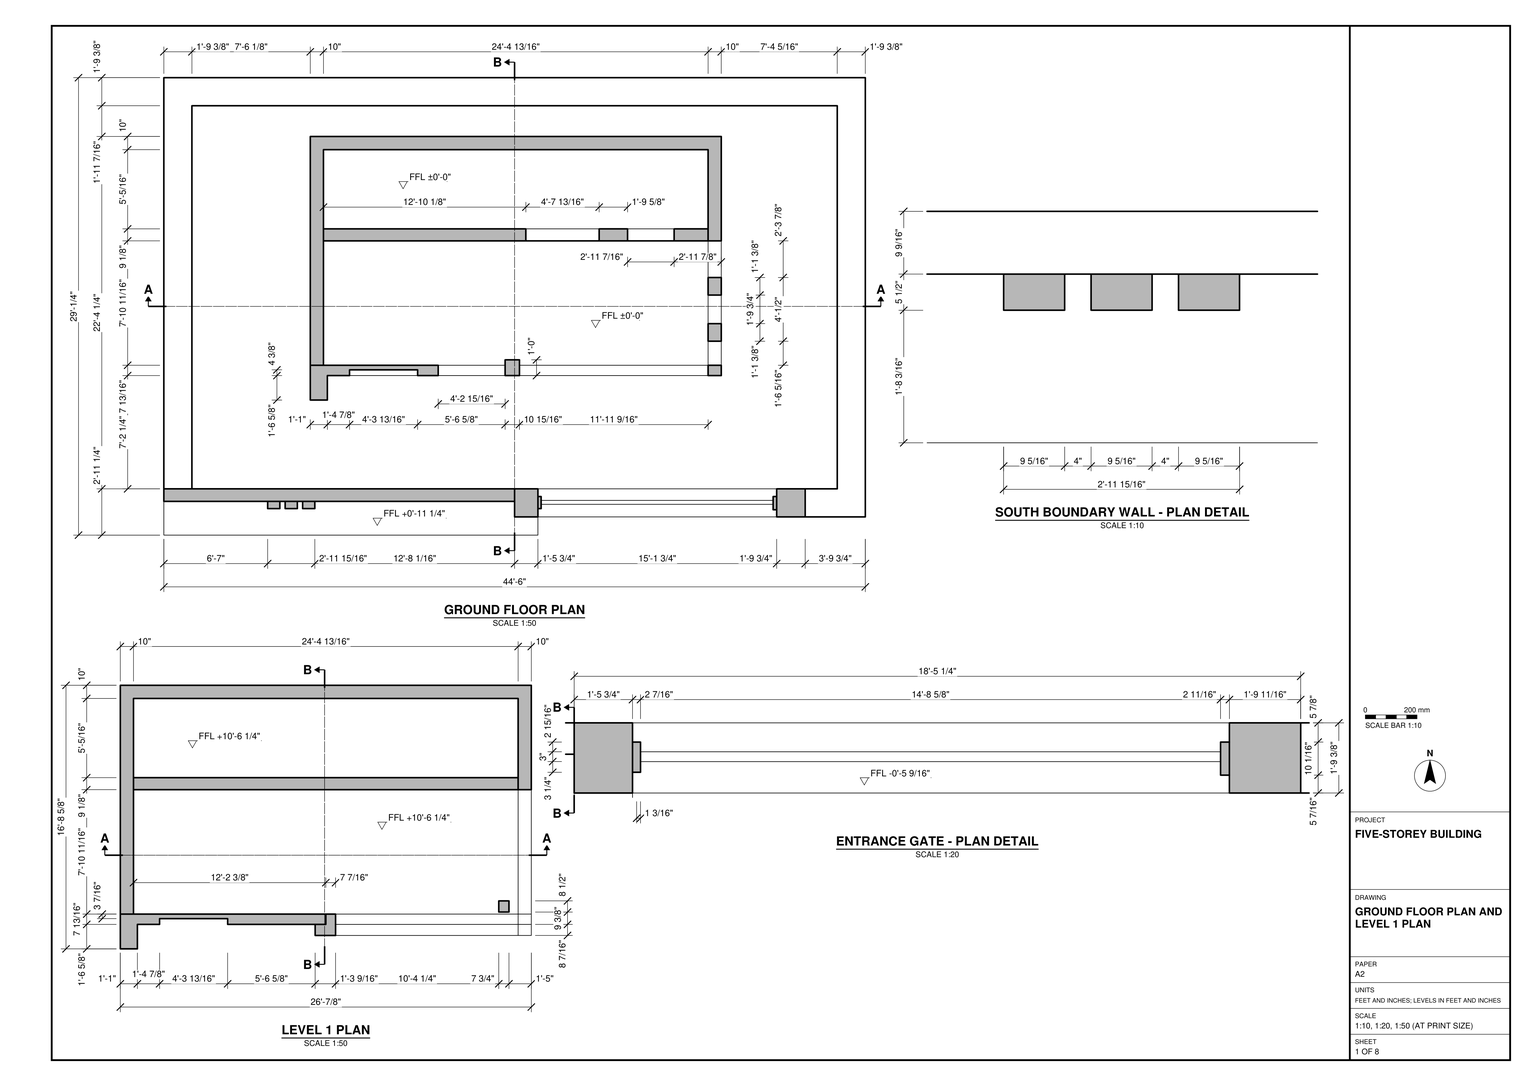
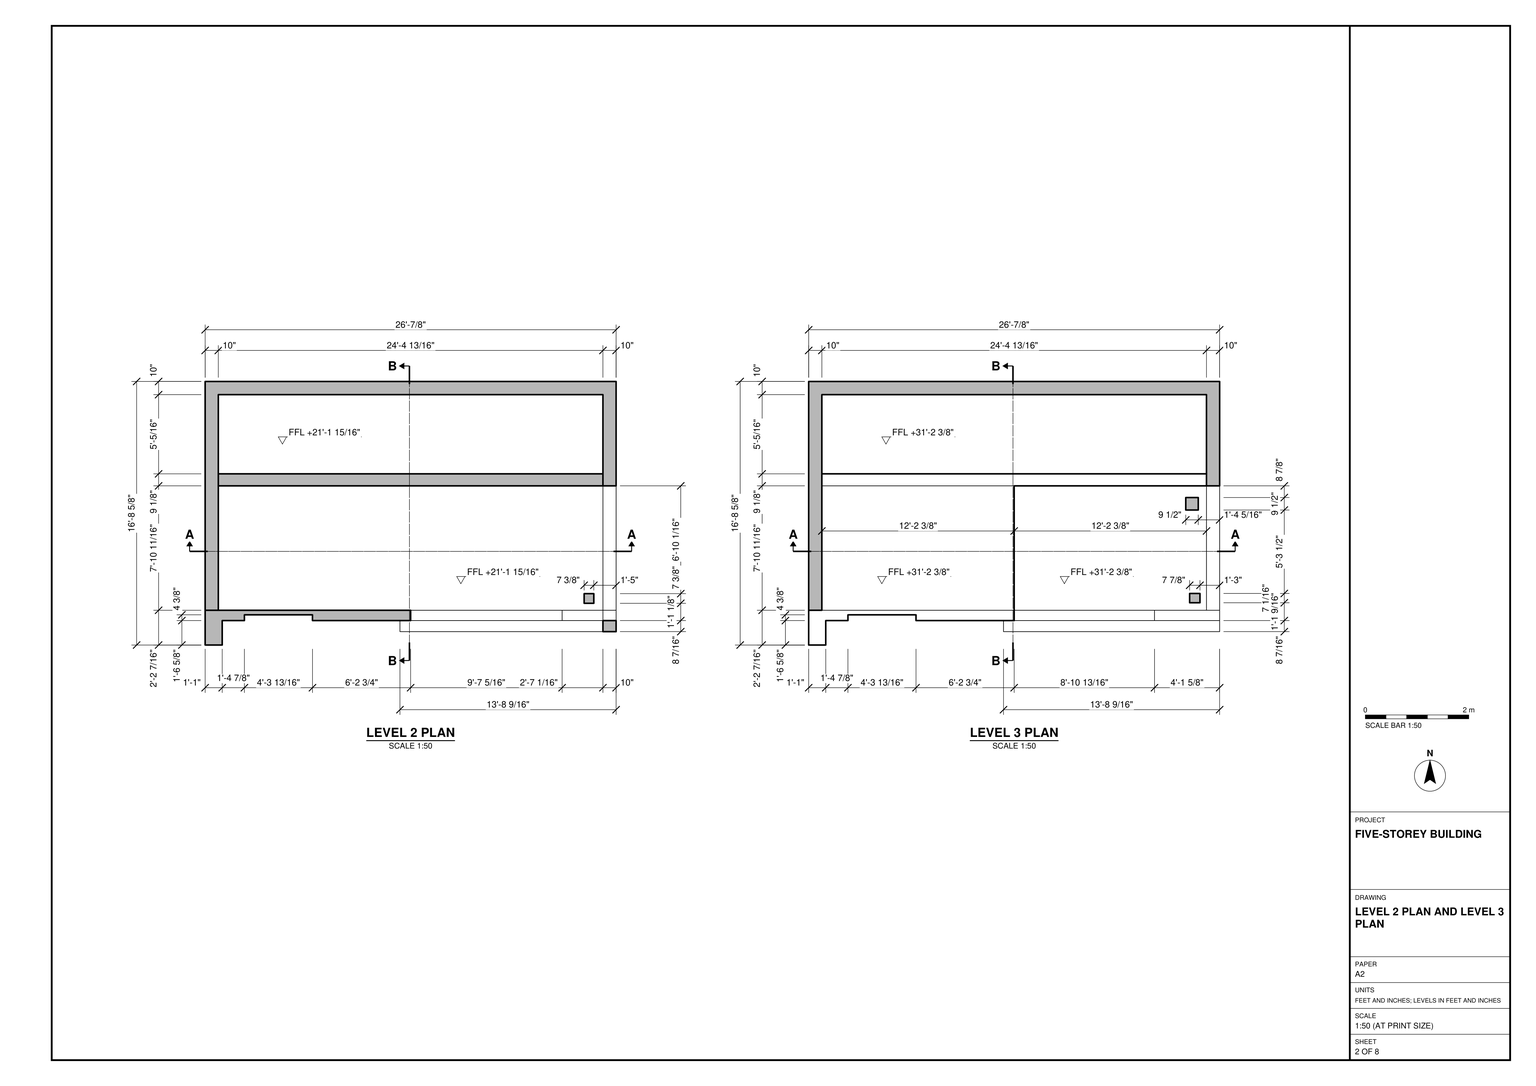
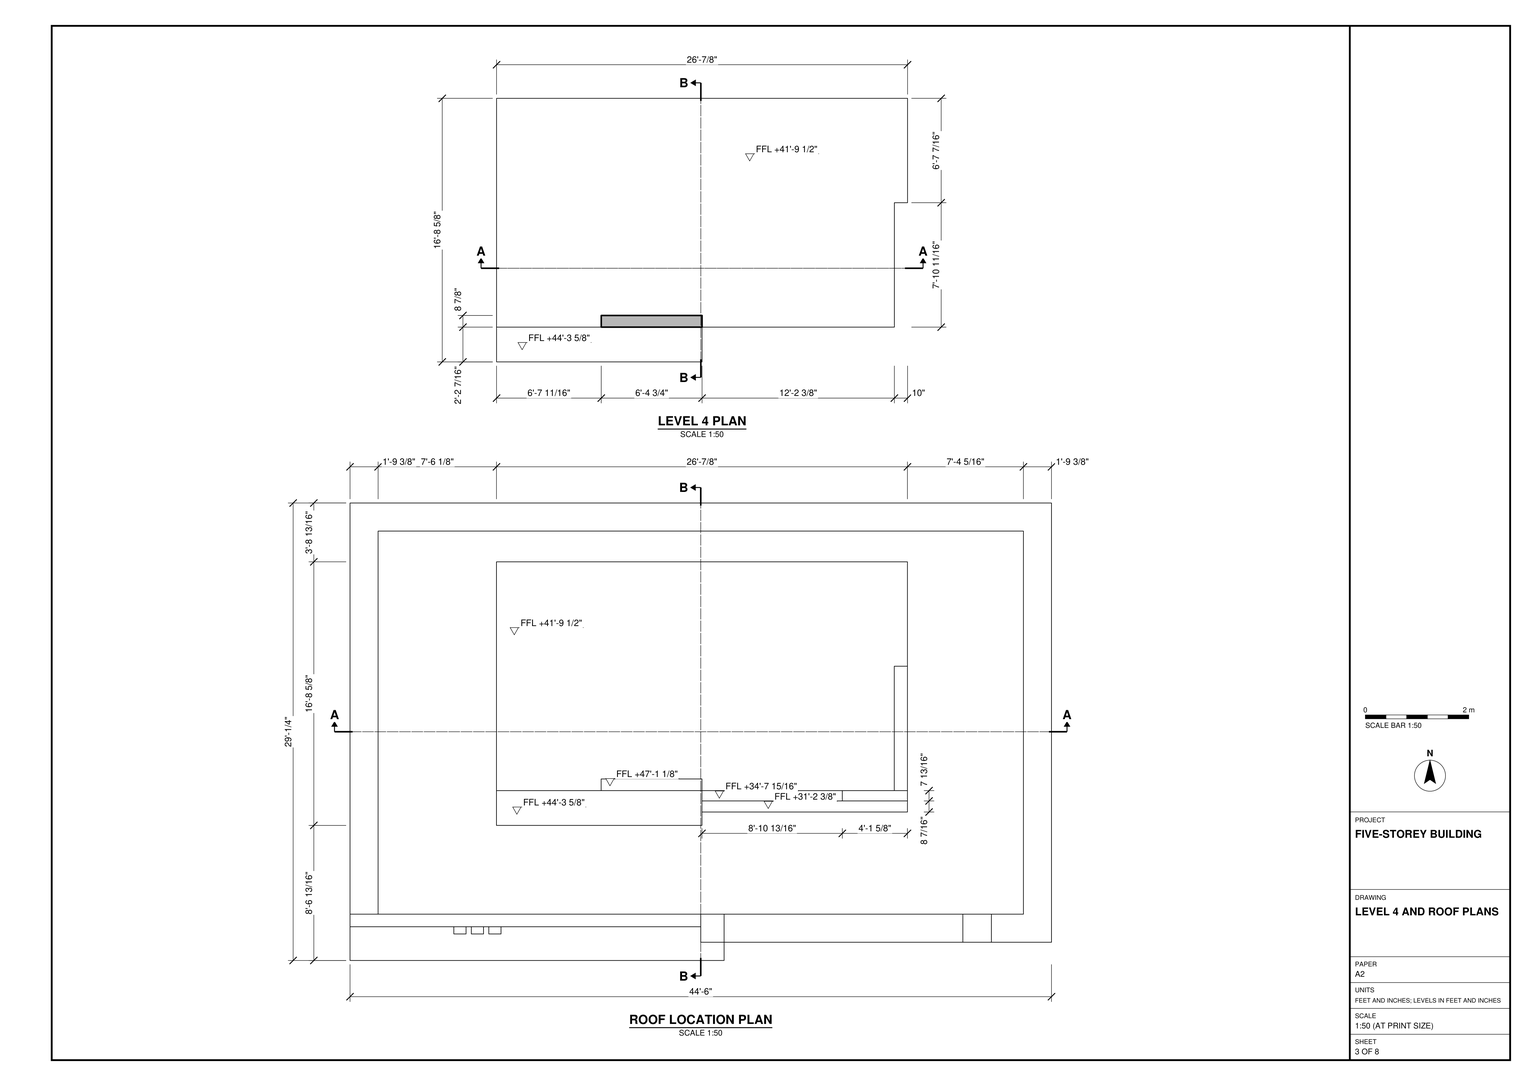
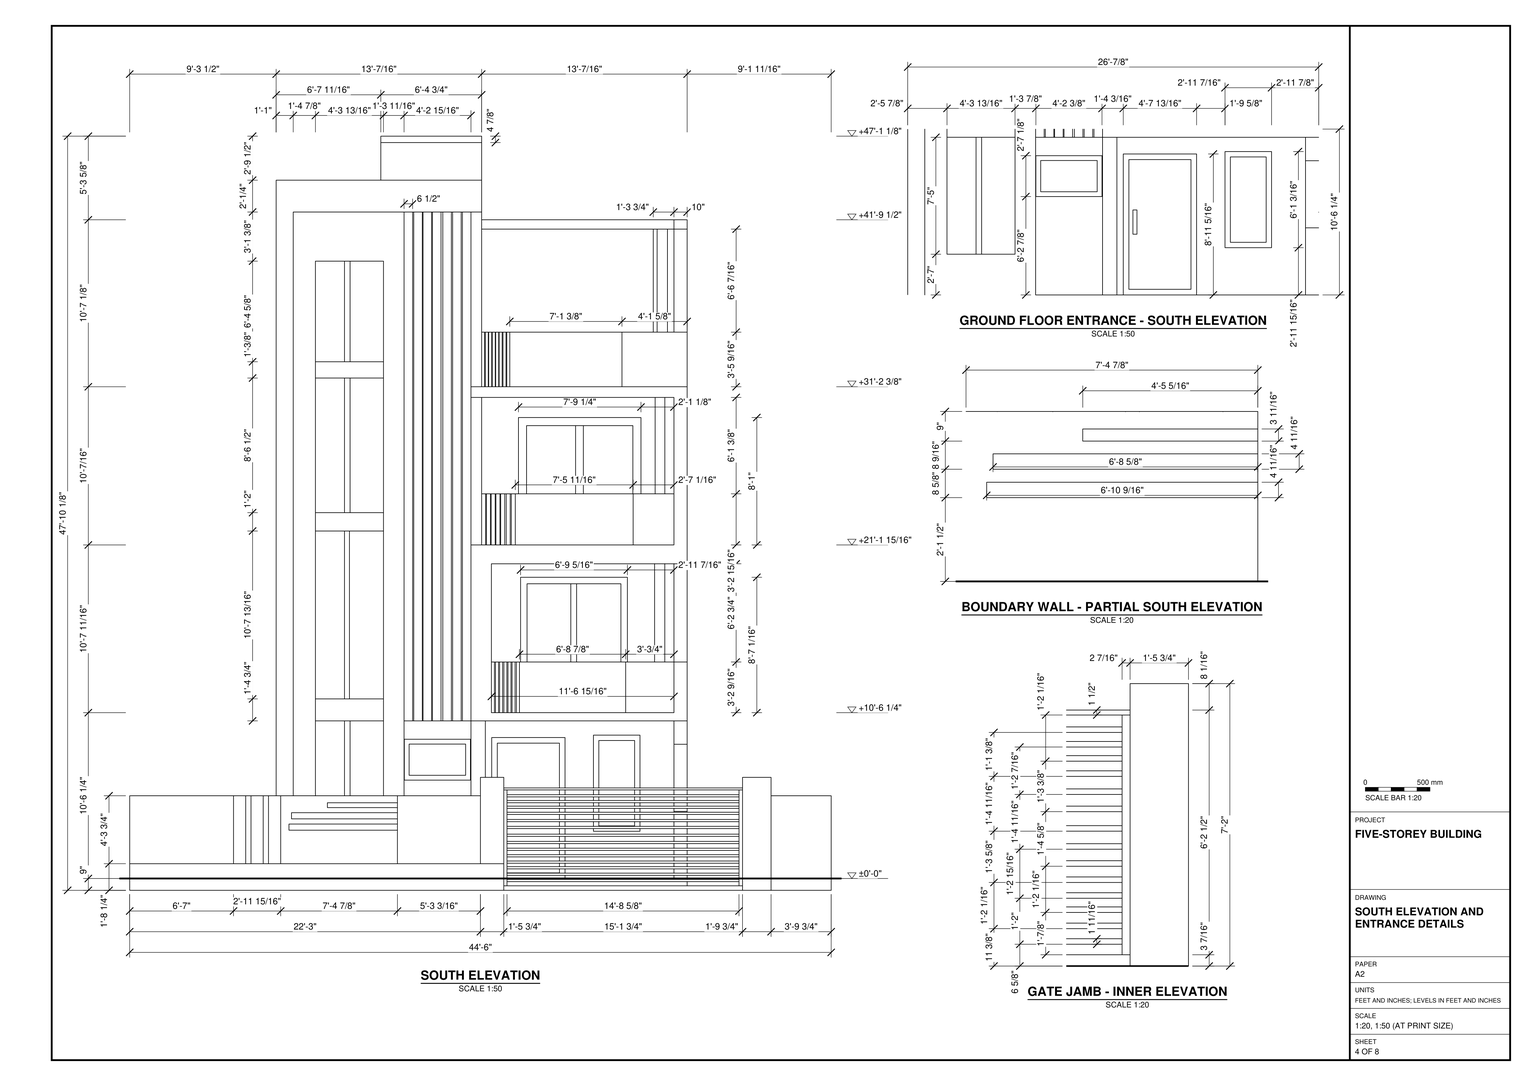
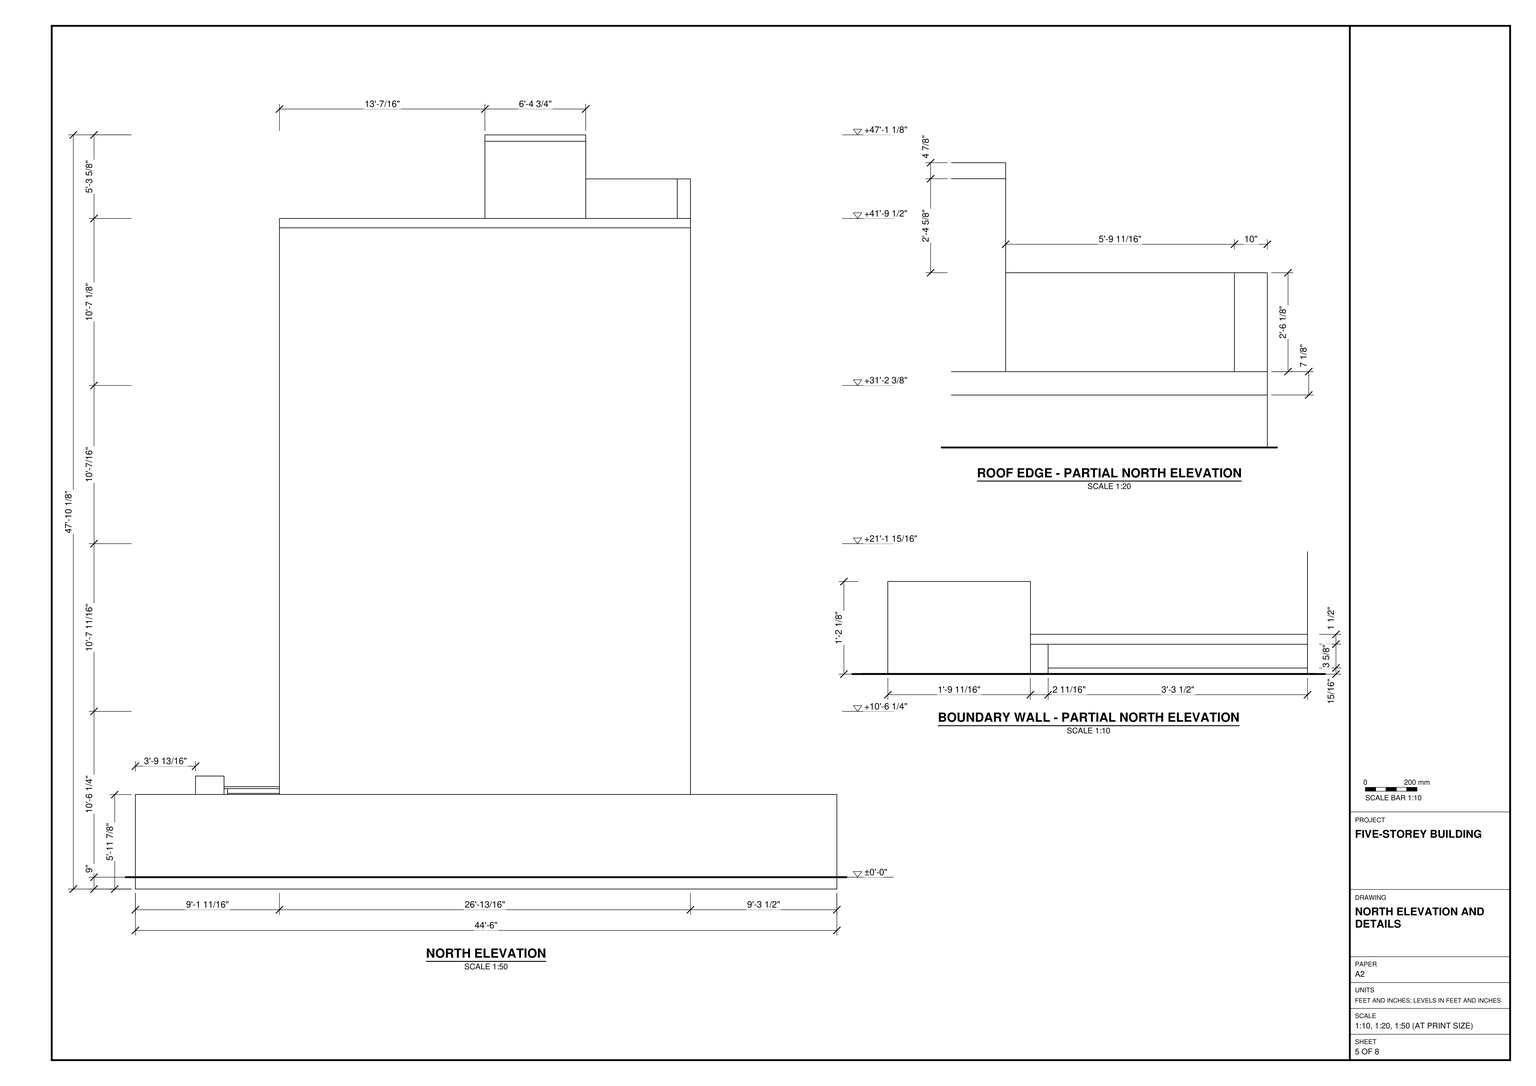
Use task_files/diagram_01.pdf to build the five-storey building and its site in SketchUp. Work in feet and inches. The complete model, including the site and gate, measures 44'-6" along X, 29'-1/4" along Y and 47'-10 1/8" along Z. Set the finished floor levels to ±0'-0", +10'-6 1/4", +21'-1 15/16", +31'-2 3/8" and +41'-9 1/2", in order from the ground floor to level 4.

Use the ground floor and roof location plans to set out the building within the site, leaving more space on the entrance side than at the rear. Model the south boundary wall, its three small projections and the gate between its posts. Follow each floor plan for wall thicknesses, including the 10" rear wall, and distinguish the narrow rear bay from the deeper space in front. Match the wall openings, stepped southwest frontage, exposed slab edges and square supports to their respective plans. Use the level 4 and roof plans to shape the flat roof, including the jog in its east edge and the raised portions along its south edge.

Model stairs, built-in joinery and main furniture where shown. Keep walls, slabs, roof elements and each furniture or joinery piece in separate groups or components, and use components for repeated parts. Any decor or loose items shown may be represented by suitable library components. Save one SketchUp model as output_files/five_storey_building_with_its_gated_south_frontage.skp.

# SketchUp Ruby script. Lengths in inches.
U = 1.inch
M = Sketchup.active_model
def pt(a) = Geom::Point3d.new(a.map { |v| v * U })
def face(e, loops, mat)
  f = e.add_face(loops[0].map { |a| pt(a) })
  loops[1..].each { |l| e.add_face(l.map { |a| pt(a) }).erase! }
  f.material = f.back_material = mat if mat
  f
end
# faces: each face lists its corners as indices into pts; further lists are holes
def faces(e, pts, list, mat = nil) = list.each { |f| face(e, (f[0].is_a?(Array) ? f : [f]).map { |l| l.map { |i| pts[i] } }, mat) }
# xy, xz, yz: faces in a plane at the given z, y or x. An outline is a flat list of corners, or four numbers for a rectangle; further outlines are holes
def ring(l) = l.size == 4 ? [[l[0], l[1]], [l[2], l[1]], [l[2], l[3]], [l[0], l[3]]] : l.each_slice(2).to_a
def flat(e, list, mat, &to3) = list.each { |f| face(e, (f[0].is_a?(Array) ? f : [f]).map { |l| ring(l).map { |u, v| to3.(u, v) } }, mat) }
def xy(e, z, list, mat = nil) = flat(e, list, mat) { |x, y| [x, y, z] }
def xz(e, y, list, mat = nil) = flat(e, list, mat) { |x, z| [x, y, z] }
def yz(e, x, list, mat = nil) = flat(e, list, mat) { |y, z| [x, y, z] }
def lines(e, pts, list) = list.each { |a, b| e.add_line(pt(pts[a]), pt(pts[b])) }
# prism: a flat outline (further loops are holes) pulled along v
def prism(e, loops, v, mat = nil)
  f = face(e, loops, mat); d = Geom::Vector3d.new(v.map { |x| x * U })
  f.pushpull(f.normal.samedirection?(d) ? d.length : -d.length)
end
def box(e, o, s, mat = nil) = prism(e, [[o, [o[0] + s[0], o[1], o[2]], [o[0] + s[0], o[1] + s[1], o[2]], [o[0], o[1] + s[1], o[2]]]], [0, 0, s[2]], mat)
def at(x, y, z, deg = 0) = Geom::Transformation.translation(pt([x, y, z])) * Geom::Transformation.rotation(ORIGIN, Z_AXIS, deg.degrees)
def axes(o, x, y, z) = Geom::Transformation.new([*x, 0, *y, 0, *z, 0, *pt(o).to_a, 1])
def part(name) = M.definitions.add(name)
# library, detail: a bought-in or finely detailed component or shape, given as its bounding box
def library(name, o, s) = part(name).tap { |d| box(d.entities, o, s) }
def detail(e, o, s) = box(e.add_group.entities, o, s)
def put(e, d, t, mat = nil) = e.add_instance(d, t).tap { |i| i.material = mat if mat }
def group(e, t, mat = nil) = e.add_group.tap { |g| g.transformation = t; g.material = mat if mat }.entities
root = M.entities
M.materials.add("[0006_Pink]").color = [255, 192, 203]
M.materials.add("[0012_Bisque]").color = [229, 205, 176]
M.materials.add("[Blinds Cloth Horizontal]").color = [192, 163, 85]
M.materials.add("[Color A01]").color = [255, 204, 204]
M.materials.add("[Color A08]").color = [102, 0, 0]
M.materials.add("[Color B02]").color = [255, 178, 153]
M.materials.add("[Color C01]").color = [255, 229, 204]
M.materials.add("[Color C02]").color = [255, 204, 153]
M.materials.add("[Color M08]").color = [30, 30, 30]
M.materials.add("[Concrete Pavers Block Multi]").color = [124, 140, 145]
M.materials.add("[Encaustic Tile Circular 02]").color = [187, 174, 162]
M.materials.add("[Field Square Tile]").color = [217, 201, 169]
M.materials.add("[Formica Beige]").color = [211, 187, 149]
M.materials.add("[Formica Graystone]").color = [211, 207, 191]
M.materials.add("[Formica Graystone]1").color = [149, 146, 135]
M.materials.add("[Formica Laminate Dark]").color = [50, 53, 60]
M.materials.add("[Formica Laminate Light]").color = [213, 189, 164]
M.materials.add("[Formica Speckled Grey]").color = [94, 105, 111]
M.materials.add("[Pavers Flagstone Gray]").color = [162, 162, 162]
M.materials.add("[Quartz Light Brown]").color = [199, 184, 152]
M.materials.add("[Terrazzo Tile Light]").color = [219, 217, 210]
M.materials.add("[Tile Limestone Large]").color = [238, 251, 230]
M.materials.add("[Tile Limestone Multi]").color = [199, 173, 118]
M.materials.add("[Tile Various Tan]").color = [214, 196, 169]
M.materials.add("[Translucent Glass Gray]").color = [128, 128, 128]
M.materials["[Translucent Glass Gray]"].alpha = 0.5
M.materials.add("[Translucent Glass Safety]").color = [204, 235, 244]
M.materials["[Translucent Glass Safety]"].alpha = 0.5
M.materials.add("[Window Covering 02]").color = [255, 228, 147]
M.materials.add("[Window Covering 02]1").color = [239, 214, 138]
M.materials.add("[Wood Bamboo]").color = [177, 105, 43]
M.materials.add("[Wood Cherry Original]").color = [152, 86, 42]
M.materials.add("[Wood Floor Light]").color = [204, 176, 127]
M.materials.add("[Wood Veneer 01]").color = [120, 70, 37]
xy(root,0,[[0,0,0,35.24,267,35.24,267,13.875,284.77,13.875,284.77,0],[488.24,13.875,488.24,35.24,512.63,35.24,512.63,326.9,21.37,326.9,21.37,35.24,0,35.24,0,348.27,534,348.27,534,13.875],[267,13.875,284.77,35.24],[284.77,13.875,466.52,35.24],[466.52,13.875,488.24,35.24],
  [111.48,102.84,111.48,303.48,424.34,303.48,424.34,121.46,124.48,121.46,124.48,102.84]])
xy(root,0,[[[21.37,35.24,512.63,326.9],[111.48,102.84,124.48,102.84,124.48,121.46,424.34,121.46,424.34,303.48,111.48,303.48]]],"[Pavers Flagstone Gray]")
xy(root,3.4375,[[463.83,19.32,466.52,29.39],[284.77,20.19,287.21,29.39]])
xy(root,3.4375,[[284.77,13.875,466.52,13.875,466.52,19.32,463.83,19.32,463.83,29.39,466.52,29.39,466.52,35.24,284.77,35.24,284.77,29.39,287.21,29.39,287.21,20.19,284.77,20.19]],"[Color M08]")
xy(root,6.63,[[287.21,23.43,463.83,26.43]])
xy(root,8.32,[[287.21,23.43,463.83,26.43]],"[Formica Laminate Dark]")
xy(root,9,[[259.79,121.46,270.73,129.3],[414.31,121.46,424.34,129.3],[111.48,129.3,111.48,303.48,424.34,303.48,424.34,224.02,414.31,224.02,414.31,293.45,121.51,293.45,121.51,129.3],[259.79,129.3,270.73,133.46],[414.31,147.64,424.34,161],
  [414.31,182.76,424.34,196.13],[121.51,224.02,275.57,233.16],[275.57,224.02,331.39,233.16],[331.39,224.02,414.31,233.16],[121.51,233.16,414.31,293.45]])
xy(root,9,[[208.86,121.46,259.79,129.3],[270.73,121.46,414.31,129.3],[121.51,129.3,259.79,129.3,259.79,133.46,270.73,133.46,270.73,129.3,414.31,129.3,414.31,224.02,121.51,224.02],[414.31,129.3,424.34,147.64],[414.31,161,424.34,182.76],
  [414.31,196.13,424.34,224.02]],"[Field Square Tile]")
xy(root,11.38,[[287.21,23.43,463.83,26.43]])
xy(root,13.07,[[287.21,23.43,463.83,26.43]],"[Formica Laminate Dark]")
xy(root,16.32,[[287.21,23.43,463.83,26.43]])
xy(root,18.01,[[287.21,23.43,463.83,26.43]],"[Formica Laminate Dark]")
xy(root,20.25,[[79.03,20.1875,88.32,25.6875],[92.34,20.1875,101.63,25.6875],[105.65,20.1875,114.94,25.6875]])
xy(root,20.25,[[0,0,284.77,0,284.77,13.875,267,13.875,267,25.6875,114.94,25.6875,114.94,20.1875,105.65,20.1875,105.65,25.6875,101.63,25.6875,101.63,20.1875,92.34,20.1875,92.34,25.6875,88.32,25.6875,88.32,20.1875,79.03,20.1875,79.03,25.6875,0,25.6875]],"[Color C01]")
xy(root,20.63,[[287.21,23.43,463.83,26.43]])
xy(root,22.32,[[287.21,23.43,463.83,26.43]],"[Formica Laminate Dark]")
xy(root,25.44,[[287.21,23.43,463.83,26.43]])
xy(root,27.13,[[287.21,23.43,463.83,26.43]],"[Formica Laminate Dark]")
xy(root,30.38,[[287.21,23.43,463.83,26.43]])
xy(root,32.07,[[287.21,23.43,463.83,26.43]],"[Formica Laminate Dark]")
xy(root,35.57,[[286.02,23.43,463.83,26.43]])
xy(root,37.26,[[286.02,23.43,463.83,26.43]],"[Formica Laminate Dark]")
xy(root,39.99,[[141.375,121.46,193.1875,125.84]],"[Formica Graystone]")
xy(root,41.07,[[287.21,23.43,463.83,26.43]])
xy(root,42.76,[[287.21,23.43,463.83,26.43]],"[Formica Laminate Dark]")
xy(root,44.96,[[353.02,224.02,388.45,233.16]])
xy(root,47.01,[[287.21,23.43,463.83,26.43]])
xy(root,48.69,[[287.21,23.43,463.83,26.43]],"[Formica Laminate Dark]")
xy(root,52.26,[[287.21,23.43,463.83,26.43]])
xy(root,53.94,[[287.21,23.43,463.83,26.43]],"[Formica Laminate Dark]")
xy(root,57.76,[[287.21,23.43,463.83,26.43]])
xy(root,59.44,[[287.21,23.43,463.83,26.43]],"[Formica Laminate Dark]")
xy(root,60.09,[[414.31,121.46,424.34,129.3],[414.31,147.64,424.34,161],[414.31,182.76,424.34,196.13]])
xy(root,62.38,[[287.21,23.43,463.83,26.43]])
xy(root,64.07,[[287.21,23.43,463.83,26.43]],"[Formica Laminate Dark]")
xy(root,66.69,[[287.21,23.43,463.83,26.43]])
xy(root,68.38,[[287.21,23.43,463.83,26.43]],"[Formica Laminate Dark]")
xy(root,71.13,[[287.21,23.43,463.83,26.43]])
xy(root,72,[[79.03,20.1875,88.32,25.6875],[92.34,20.1875,101.63,25.6875],[105.65,20.1875,114.94,25.6875]])
xy(root,72,[[488.24,13.875,534,13.875,534,348.27,0,348.27,0,35.24,21.37,35.24,21.37,326.9,512.63,326.9,512.63,35.24,488.24,35.24],[0,25.6875,267,35.24]],"[Tile Limestone Large]")
xy(root,72.82,[[287.21,23.43,463.83,26.43]],"[Formica Laminate Dark]")
xy(root,76.4375,[[284.77,13.875,284.77,20.19,287.21,20.19,287.21,24.69,463.83,24.69,463.83,19.32,466.52,19.32,466.52,13.875],[463.83,19.32,466.52,29.39],[284.77,20.19,287.21,29.39],[287.21,24.69,463.83,29.39],[284.77,29.39,466.52,35.24]])
xy(root,77.95,[[284.77,13.875,466.52,35.24]],"[Color M08]")
xy(root,83.89,[[209.03,224.02,259.4,233.16]])
xy(root,86,[[267,13.875,284.77,35.24],[466.52,13.875,488.24,35.24]],"[Color C01]")
xy(root,111.18,[[414.31,121.46,424.34,129.3],[414.31,147.64,424.34,161],[414.31,182.76,424.34,196.13]])
xy(root,115.01,[[209.03,224.02,259.4,233.16]])
xy(root,116.3125,[[275.57,224.02,331.39,233.16]])
xy(root,118.15,[[353.02,224.02,388.45,233.16]])
xy(root,129,[[259.79,121.46,270.73,133.46],[414.31,121.46,424.34,129.3],[414.31,129.3,424.34,147.64],[414.31,147.64,424.34,161],[414.31,182.76,424.34,196.13],
  [121.51,224.02,414.31,233.16],[121.51,233.16,414.31,293.45]])
xy(root,129,[[259.79,113.02,414.31,121.46],[414.31,113.02,424.34,121.46]],"[0006_Pink]")
xy(root,129,[[208.86,121.46,208.86,129.3,121.51,129.3,121.51,224.02,424.34,224.02,424.34,196.13,414.31,196.13,414.31,182.76,424.34,182.76,424.34,161,414.31,161,414.31,121.46,270.73,121.46,270.73,133.46,259.79,133.46,259.79,121.46]],"[Color C02]")
xy(root,131.0625,[[259.79,121.46,270.73,133.46]])
xy(root,135.25,[[399.59,130.85,407.34,139.35],[121.51,224.02,414.31,233.16],[121.51,233.16,414.31,293.45]])
xy(root,135.25,[[275.34,113.02,414.31,121.46]],"[0006_Pink]")
xy(root,135.25,[[[121.51,129.3,414.31,224.02],[399.59,130.85,407.34,139.35]]],"[Tile Limestone Multi]")
xy(root,173.8125,[[414.31,113.02,424.34,121.46]],"[0006_Pink]")
xy(root,173.8125,[[275.34,121.46,414.31,129.3],[414.31,121.46,424.34,129.3]],"[Formica Beige]")
xy(root,173.8125,[[414.31,129.3,424.34,224.02]],"[Translucent Glass Safety]")
xy(root,248.58,[[275.34,113.02,424.34,129.3]],"[Color A01]")
xy(root,255.25,[[121.51,224.02,414.31,233.16],[121.51,233.16,414.31,293.45]])
xy(root,255.25,[[[121.51,129.3,424.34,224.02],[399.59,130.85,407.34,139.35]]],"[Color C02]")
xy(root,262.9375,[[267.92,121.46,414.31,129.3],[414.31,121.46,424.34,129.3],[414.31,129.3,424.34,224.02],[399.99,134.6,407.37,141.97],[121.51,224.02,414.31,233.16],
  [121.51,233.16,414.31,293.45]])
xy(root,262.9375,[[259.79,113.02,414.31,121.46]],"[0006_Pink]")
xy(root,262.9375,[[[121.51,129.3,414.31,224.02],[399.99,134.6,407.37,141.97]]],"[Encaustic Tile Circular 02]")
xy(root,301.875,[[383.24,121.46,414.31,129.3],[414.31,121.46,424.34,129.3]],"[Formica Laminate Dark]")
xy(root,301.875,[[267.92,121.46,383.24,129.3],[414.31,129.3,424.34,224.02]],"[Translucent Glass Safety]")
xy(root,375.25,[[121.51,224.02,414.31,233.16],[121.51,233.16,414.31,293.45]])
xy(root,375.25,[[[259.79,113.02,259.79,121.46,267.92,121.46,267.92,129.3,121.51,129.3,121.51,224.02,424.34,224.02,424.34,121.46,414.31,121.46,414.31,113.02],[399.99,134.6,407.37,141.97]]],"[Color C02]")
xy(root,383.375,[[414.31,121.46,424.34,224.02],[121.51,129.3,267.92,224.02],[401.49,135.03,409.36,142.09],[398.55,205.62,408.05,215.12],[121.51,224.02,414.31,233.16],
  [121.51,233.16,414.31,293.45]])
xy(root,383.375,[[259.79,113.02,424.34,121.46]],"[0006_Pink]")
xy(root,383.375,[[[267.92,129.3,414.31,224.02],[398.55,205.62,408.05,215.12],[401.49,135.03,409.36,142.09]]],"[Concrete Pavers Block Multi]")
xy(root,424.9375,[[374.74,121.46,424.34,129.3]],"[Formica Beige]")
xy(root,424.9375,[[267.92,121.46,374.74,129.3],[414.31,129.3,424.34,224.02]],"[Translucent Glass Safety]")
xy(root,478.99,[[141.375,121.46,193.1875,125.84]],"[Formica Graystone]")
xy(root,503.375,[[111.48,129.3,121.51,224.02],[121.51,129.3,267.92,224.02],[303.23,147.13,301.65,147.34,300.17,147.95,298.9,148.92,297.93,150.19,297.3125,151.67,297.11,153.25,297.3125,154.84,297.93,156.32,298.9,157.58,300.17,158.56,301.65,159.17,303.23,159.38,304.82,159.17,306.29,158.56,307.5625,157.58,308.54,156.32,309.15,154.84,309.36,153.25,309.15,151.67,308.54,150.19,307.5625,148.92,306.29,147.95,304.82,147.34],[363.04,147.13,361.46,147.34,359.98,147.95,358.71,148.92,357.74,150.19,357.125,151.67,356.92,153.25,357.125,154.84,357.74,156.32,358.71,157.58,359.98,158.56,361.46,159.17,363.04,159.38,364.63,159.17,366.11,158.56,367.375,157.58,368.35,156.32,368.96,154.84,369.17,153.25,368.96,151.67,368.35,150.19,367.375,148.92,366.11,147.95,364.63,147.34],[300.98,193.94,299.4,194.15,297.92,194.76,296.65,195.73,295.68,197,295.0625,198.48,294.86,200.07,295.0625,201.65,295.68,203.13,296.65,204.4,297.92,205.37,299.4,205.98,300.98,206.19,302.57,205.98,304.04,205.37,305.3125,204.4,306.29,203.13,306.9,201.65,307.11,200.07,306.9,198.48,306.29,197,305.3125,195.73,304.04,194.76,302.57,194.15],
  [363.04,193.94,361.46,194.15,359.98,194.76,358.71,195.73,357.74,197,357.125,198.48,356.92,200.07,357.125,201.65,357.74,203.13,358.71,204.4,359.98,205.37,361.46,205.98,363.04,206.19,364.63,205.98,366.11,205.37,367.375,204.4,368.35,203.13,368.96,201.65,369.17,200.07,368.96,198.48,368.35,197,367.375,195.73,366.11,194.76,364.63,194.15],[111.48,224.02,121.51,233.16],[121.51,224.02,414.31,233.16],[414.31,224.02,424.34,233.16],[111.48,233.16,121.51,293.45],
  [121.51,233.16,414.31,293.45],[414.31,233.16,424.34,303.48],[111.48,293.45,414.31,303.48]])
xy(root,503.375,[[[267.92,129.3,414.31,224.02],[303.23,147.13,304.82,147.34,306.29,147.95,307.5625,148.92,308.54,150.19,309.15,151.67,309.36,153.25,309.15,154.84,308.54,156.32,307.5625,157.58,306.29,158.56,304.82,159.17,303.23,159.38,301.65,159.17,300.17,158.56,298.9,157.58,297.93,156.32,297.3125,154.84,297.11,153.25,297.3125,151.67,297.93,150.19,298.9,148.92,300.17,147.95,301.65,147.34],[363.04,147.13,364.63,147.34,366.11,147.95,367.375,148.92,368.35,150.19,368.96,151.67,369.17,153.25,368.96,154.84,368.35,156.32,367.375,157.58,366.11,158.56,364.63,159.17,363.04,159.38,361.46,159.17,359.98,158.56,358.71,157.58,357.74,156.32,357.125,154.84,356.92,153.25,357.125,151.67,357.74,150.19,358.71,148.92,359.98,147.95,361.46,147.34],[363.04,193.94,364.63,194.15,366.11,194.76,367.375,195.73,368.35,197,368.96,198.48,369.17,200.07,368.96,201.65,368.35,203.13,367.375,204.4,366.11,205.37,364.63,205.98,363.04,206.19,361.46,205.98,359.98,205.37,358.71,204.4,357.74,203.13,357.125,201.65,356.92,200.07,357.125,198.48,357.74,197,358.71,195.73,359.98,194.76,361.46,194.15],[300.98,193.94,302.57,194.15,304.04,194.76,305.3125,195.73,306.29,197,306.9,198.48,307.11,200.07,306.9,201.65,306.29,203.13,305.3125,204.4,304.04,205.37,302.57,205.98,300.98,206.19,299.4,205.98,297.92,205.37,296.65,204.4,295.68,203.13,295.0625,201.65,294.86,200.07,295.0625,198.48,295.68,197,296.65,195.73,297.92,194.76,299.4,194.15],[398.55,205.62,408.05,215.12],[401.49,135.03,409.36,142.09]]],"[Wood Veneer 01]")
xy(root,510.5,[[191.17,129.3,267.92,138.18]])
xy(root,510.5,[[111.48,129.3,191.17,129.3,191.17,138.18,267.92,138.18,267.92,129.3,414.31,129.3,414.31,224.02,424.34,224.02,424.34,303.48,111.48,303.48]],"[Formica Graystone]1")
xy(root,516.39,[[124.48,102.84,267.92,121.46]],"[Terrazzo Tile Light]")
xy(root,540.625,[[111.48,102.84,267.92,129.3]],"[Terrazzo Tile Light]")
xy(root,569.25,[[191.17,129.3,267.92,138.18]])
xy(root,574.125,[[191.17,129.3,267.92,138.18]],"[Formica Graystone]1")
xz(root,0,[[0,0,284.77,20.25]],"[Color C01]")
xz(root,13.875,[[267,0,284.77,20.25]])
xz(root,13.875,[[466.52,0,488.24,86],[488.24,0,534,72],[267,20.25,284.77,86]],"[Color C01]")
xz(root,13.875,[[284.77,0,466.52,3.4375],[284.77,76.4375,466.52,77.95]],"[Color M08]")
xz(root,19.32,[[463.83,3.4375,466.52,76.4375]],"[Color M08]")
xz(root,20.1875,[[79.03,20.25,88.32,72],[92.34,20.25,101.63,72],[105.65,20.25,114.94,72]])
xz(root,20.19,[[284.77,3.4375,287.21,76.4375]],"[Color M08]")
xz(root,23.43,[[287.21,6.63,463.83,8.32],[287.21,11.38,463.83,13.07],[287.21,16.32,463.83,18.01],[287.21,20.63,463.83,22.32],[287.21,25.44,463.83,27.13],
  [287.21,30.38,463.83,32.07],[286.02,35.57,463.83,37.26],[287.21,41.07,463.83,42.76],[287.21,47.01,463.83,48.69],[287.21,52.26,463.83,53.94],
  [287.21,57.76,463.83,59.44],[287.21,62.38,463.83,64.07],[287.21,66.69,463.83,68.38],[287.21,71.13,463.83,72.82]],"[Formica Laminate Dark]")
xz(root,25.6875,[[79.03,20.25,88.32,72],[92.34,20.25,101.63,72],[105.65,20.25,114.94,72],[121.24,45.77,203.8,50.45],[123.18,54.41,203.8,59.1],
  [150.49,62.98,203.8,66.67]])
xz(root,25.6875,[[203.8,20.25,267,72]],"[Color C01]")
xz(root,25.6875,[[0,20.25,79.03,72],[88.32,20.25,92.34,72],[101.63,20.25,105.65,72],[114.94,20.25,203.8,20.25,203.8,45.77,121.24,45.77,121.24,50.45,203.8,50.45,203.8,54.41,123.18,54.41,123.18,59.1,203.8,59.1,203.8,62.98,150.49,62.98,150.49,66.67,203.8,66.67,203.8,72,114.94,72]],"[Formica Laminate Dark]")
xz(root,26.43,[[287.21,6.63,463.83,8.32],[287.21,11.38,463.83,13.07],[287.21,16.32,463.83,18.01],[287.21,20.63,463.83,22.32],[287.21,25.44,463.83,27.13],
  [287.21,30.38,463.83,32.07],[286.02,35.57,463.83,37.26],[287.21,41.07,463.83,42.76],[287.21,47.01,463.83,48.69],[287.21,52.26,463.83,53.94],
  [287.21,57.76,463.83,59.44],[287.21,62.38,463.83,64.07],[287.21,66.69,463.83,68.38],[287.21,71.13,463.83,72.82]],"[Formica Laminate Dark]")
xz(root,29.39,[[284.77,3.4375,287.21,76.4375],[463.83,3.4375,466.52,76.4375]],"[Formica Laminate Dark]")
xz(root,35.24,[[0,0,21.37,20.25],[0,20.25,21.37,72]])
xz(root,35.24,[[267,0,284.77,86],[466.52,0,488.24,86]],"[Color C01]")
xz(root,35.24,[[284.77,0,466.52,3.4375],[284.77,76.4375,466.52,77.95]],"[Color M08]")
xz(root,35.24,[[21.37,0,267,72],[488.24,0,512.63,72]],"[Tile Limestone Large]")
xz(root,102.84,[[111.48,0,124.48,0,124.48,516.39,267.92,516.39,267.92,540.625,111.48,540.625]],"[Terrazzo Tile Light]")
xz(root,113.02,[[259.79,129,424.34,129,424.34,173.8125,414.31,173.8125,414.31,135.25,275.34,135.25,275.34,248.58,424.34,248.58,424.34,383.375,259.79,383.375,259.79,375.25,414.31,375.25,414.31,262.9375,259.79,262.9375]],"[0006_Pink]")
xz(root,121.46,[[259.79,129,270.73,131.0625],[259.79,135.25,267.92,262.9375],[414.31,262.9375,424.34,301.875],[414.31,301.875,424.34,375.25],[259.79,375.25,267.92,383.375]])
xz(root,121.46,[[259.79,9,270.73,129],[414.31,9,424.34,60.09],[414.31,111.18,424.34,129]],"[0012_Bisque]")
xz(root,121.46,[[414.31,60.09,424.34,111.18]],"[Color A08]")
xz(root,121.46,[[377.55,135.25,414.31,173.8125],[374.74,383.375,424.34,424.9375]],"[Formica Beige]")
xz(root,121.46,[[[124.48,0,424.34,0,424.34,9,208.86,9,208.86,516.39,124.48,516.39],[141.375,39.99,193.1875,478.99]]],"[Formica Graystone]")
xz(root,121.46,[[215.36,129,216.23,516.39],[222.74,129,223.29,516.39],[229.8,129,230.48,516.39],[236.99,129,238.36,516.39],[244.86,129,245.82,516.39],
  [252.33,129,253.29,516.39],[383.24,262.9375,414.31,301.875]],"[Formica Laminate Dark]")
xz(root,121.46,[[275.34,135.25,277.63,173.8125],[278.47,135.25,280.75,173.8125],[281.59,135.25,283.88,173.8125],[284.84,135.25,287.13,173.8125],[287.97,135.25,290.25,173.8125],
  [291.09,135.25,293.38,173.8125],[294.4,135.25,296.69,173.8125],[267.92,262.9375,270.97,301.875],[271.54,262.9375,274.59,301.875],[275.17,262.9375,278.22,301.875],
  [278.79,262.9375,281.84,301.875],[282.42,262.9375,285.47,301.875],[286.61,262.9375,289.65,301.875],[290.48,262.9375,293.53,301.875],[267.92,383.375,270.21,424.9375],
  [270.67,383.375,272.96,424.9375],[273.29,383.375,275.59,424.9375],[275.98,383.375,278.28,424.9375],[278.61,383.375,280.9,424.9375],[281.23,383.375,283.53,424.9375],
  [284.17,383.375,286.46,424.9375],[287.04,383.375,289.34,424.9375]],"[Formica Laminate Light]")
xz(root,121.46,[[208.86,129,215.36,516.39],[216.23,129,222.74,516.39],[223.29,129,229.8,516.39],[230.48,129,236.99,516.39],[238.36,129,244.86,516.39],
  [245.82,129,252.33,516.39],[253.29,129,259.79,516.39],[277.63,135.25,278.47,173.8125],[280.75,135.25,281.59,173.8125],[283.88,135.25,284.84,173.8125],
  [287.13,135.25,287.97,173.8125],[290.25,135.25,291.09,173.8125],[293.38,135.25,294.4,173.8125],[259.79,262.9375,267.92,375.25],[270.97,262.9375,271.54,301.875],
  [274.59,262.9375,275.17,301.875],[278.22,262.9375,278.79,301.875],[281.84,262.9375,282.42,301.875],[285.47,262.9375,286.61,301.875],[289.65,262.9375,290.48,301.875],
  [259.79,383.375,267.92,516.39],[270.21,383.375,270.67,424.9375],[272.96,383.375,273.29,424.9375],[275.59,383.375,275.98,424.9375],[278.28,383.375,278.61,424.9375],
  [280.9,383.375,281.23,424.9375],[283.53,383.375,284.17,424.9375],[286.46,383.375,287.04,424.9375]],"[Formica Speckled Grey]")
xz(root,121.46,[[296.69,135.25,377.55,173.8125],[293.53,262.9375,383.24,301.875],[289.34,383.375,374.74,424.9375]],"[Translucent Glass Safety]")
xz(root,125.84,[[141.375,129.02,193.1875,145.72],[141.375,273.54,193.1875,287.51],[141.375,390.01,193.1875,402.39]],"[Formica Laminate Dark]")
xz(root,125.84,[[163.5,39.99,167.76,129.02],[163.5,145.72,167.28,273.54],[163.5,287.51,167.76,390.01],[163.5,402.39,167.76,478.99]],"[Formica Speckled Grey]")
xz(root,125.84,[[141.375,39.99,163.5,129.02],[167.76,39.99,193.1875,129.02],[141.375,145.72,163.5,273.54],[167.28,145.72,193.1875,273.54],[141.375,287.51,163.5,390.01],
  [167.76,287.51,193.1875,390.01],[141.375,402.39,163.5,478.99],[167.76,402.39,193.1875,478.99]],"[Translucent Glass Safety]")
xz(root,129.3,[[111.48,9,121.51,503.375],[121.51,129,208.86,135.25],[275.34,248.58,424.34,255.25],[121.51,255.25,267.92,262.9375],[267.92,255.25,275.34,262.9375],
  [275.34,255.25,424.34,262.9375],[267.92,262.9375,275.34,301.875],[383.24,262.9375,414.31,301.875],[414.31,262.9375,424.34,301.875],[121.51,375.25,267.92,383.375],
  [111.48,503.375,121.51,510.5],[121.51,503.375,267.92,510.5],[191.17,510.5,267.92,540.625]])
xz(root,129.3,[[414.31,9,424.34,60.09],[414.31,111.18,424.34,129]],"[0012_Bisque]")
xz(root,129.3,[[414.31,60.09,424.34,111.18]],"[Color A08]")
xz(root,129.3,[[121.51,135.25,267.92,255.25],[121.51,262.9375,267.92,375.25]],"[Color B02]")
xz(root,129.3,[[121.51,9,208.86,129]],"[Color C02]")
xz(root,129.3,[[374.74,383.375,414.31,424.9375]],"[Formica Beige]")
xz(root,129.3,[[191.17,540.625,267.92,569.25],[191.17,569.25,267.92,574.125]],"[Formica Graystone]1")
xz(root,129.3,[[111.48,510.5,121.51,540.625],[121.51,510.5,191.17,540.625]],"[Terrazzo Tile Light]")
xz(root,129.3,[[267.92,135.25,267.92,255.25,275.34,255.25,275.34,173.8125,414.31,173.8125,414.31,135.25],[275.34,262.9375,383.24,301.875],[267.92,383.375,374.74,424.9375]],"[Translucent Glass Safety]")
xz(root,129.3,[[267.92,503.375,414.31,510.5]],"[Wood Veneer 01]")
xz(root,130.85,[[399.59,135.25,407.34,255.25]],"[0012_Bisque]")
xz(root,133.46,[[259.79,129,270.73,131.0625]])
xz(root,133.46,[[259.79,9,270.73,129]],"[0012_Bisque]")
xz(root,134.6,[[399.99,262.9375,407.37,375.25]],"[0012_Bisque]")
xz(root,135.03,[[401.49,383.375,409.36,503.375]],"[0012_Bisque]")
xz(root,138.18,[[191.17,510.5,267.92,569.25],[191.17,569.25,267.92,574.125]],"[Formica Graystone]1")
xz(root,139.35,[[399.59,135.25,407.34,255.25]],"[0012_Bisque]")
xz(root,141.97,[[399.99,262.9375,407.37,375.25]],"[0012_Bisque]")
xz(root,142.09,[[401.49,383.375,409.36,503.375]],"[0012_Bisque]")
xz(root,147.64,[[414.31,9,424.34,60.09],[414.31,111.18,424.34,129]],"[0012_Bisque]")
xz(root,147.64,[[414.31,60.09,424.34,111.18]],"[Color A08]")
xz(root,161,[[414.31,9,424.34,60.09],[414.31,111.18,424.34,129]],"[0012_Bisque]")
xz(root,161,[[414.31,60.09,424.34,111.18]],"[Color A08]")
xz(root,182.76,[[414.31,9,424.34,60.09],[414.31,111.18,424.34,129]],"[0012_Bisque]")
xz(root,182.76,[[414.31,60.09,424.34,111.18]],"[Color A08]")
xz(root,196.13,[[414.31,9,424.34,60.09],[414.31,111.18,424.34,129]],"[0012_Bisque]")
xz(root,196.13,[[414.31,60.09,424.34,111.18]],"[Color A08]")
xz(root,205.62,[[398.55,383.375,408.05,503.375]],"[Quartz Light Brown]")
xz(root,215.12,[[398.55,383.375,408.05,503.375]],"[Quartz Light Brown]")
xz(root,224.02,[[121.51,129,424.34,129,424.34,173.8125,414.31,173.8125,414.31,135.25,121.51,135.25],[121.51,255.25,414.31,262.9375],[414.31,255.25,424.34,262.9375],[414.31,262.9375,424.34,301.875],[121.51,375.25,414.31,383.375],
  [414.31,375.25,424.34,383.375],[414.31,383.375,424.34,424.9375]])
xz(root,224.02,[[175.58,186.28,196.33,233.78],[200.07,186.28,223.08,233.78],[169.96,310.24,188.12,354.4],[191.39,310.24,210.68,354.4]],"[Blinds Cloth Horizontal]")
xz(root,224.02,[[[121.51,9,275.57,9,275.57,116.3125,331.39,116.3125,331.39,9,414.31,9,414.31,129,121.51,129],[353.02,44.96,388.45,118.15],[209.03,83.89,259.4,115.01]],[414.31,9,424.34,129],[[121.51,135.25,297.55,135.25,297.55,238.3125,378.86,238.3125,378.86,135.25,414.31,135.25,414.31,255.25,121.51,255.25],[171.68,182.375,226.99,237.6875]],[414.31,173.8125,424.34,255.25],[[121.51,262.9375,295.95,262.9375,295.95,359.9375,389.2,359.9375,389.2,262.9375,414.31,262.9375,414.31,375.25,121.51,375.25],[166.45,306.73,214.2,357.91]],
  [414.31,301.875,424.34,375.25]],"[Color B02]")
xz(root,224.02,[[267.92,383.375,414.31,503.375],[414.31,424.9375,424.34,503.375],[414.31,503.375,424.34,510.5]],"[Terrazzo Tile Light]")
xz(root,224.02,[[212.71,87.56,255.72,111.34]],"[Translucent Glass Safety]")
xz(root,224.02,[[302.47,140.18,335.79,233.38],[340.21,140.18,373.93,233.38],[302.11,269.1,339.43,353.78],[345.34,269.1,383.04,353.78]],"[Window Covering 02]")
xz(root,224.02,[[357.11,49.05,384.36,114.06]],"[Window Covering 02]1")
xz(root,224.02,[[[275.57,9,331.39,116.3125],[279.84,13.27,327.12,112.05]],[[171.68,182.375,226.99,237.6875],[175.58,186.28,223.08,233.78]],[196.33,186.28,200.07,233.78],[[166.45,306.73,214.2,357.91],[169.96,310.24,210.68,354.4]],[188.12,310.24,191.39,354.4]],"[Wood Bamboo]")
xz(root,224.02,[[[279.84,13.27,327.12,112.05],[282.93,55.21,285.99,73.71]],[[353.02,44.96,388.45,118.15],[357.11,49.05,384.36,114.06]],[[209.03,83.89,259.4,115.01],[212.71,87.56,255.72,111.34]]],"[Wood Cherry Original]")
xz(root,224.02,[[282.93,55.21,285.99,73.71]],"[Wood Floor Light]")
xz(root,224.02,[[[297.55,135.25,378.86,238.3125],[302.47,140.18,373.93,233.38]],[335.79,140.18,340.21,233.38],[[295.95,262.9375,389.2,359.9375],[302.11,269.1,383.04,353.78]],[339.43,269.1,345.34,353.78]],"[Wood Veneer 01]")
xz(root,233.16,[[[121.51,9,121.51,129,414.31,129,414.31,9,331.39,9,331.39,116.3125,275.57,116.3125,275.57,9],[353.02,44.96,388.45,118.15],[209.03,83.89,259.4,115.01]],[121.51,135.25,414.31,255.25],[121.51,255.25,414.31,262.9375],[121.51,262.9375,414.31,375.25],[121.51,375.25,414.31,383.375],
  [121.51,383.375,414.31,503.375]])
xz(root,293.45,[[121.51,9,414.31,129],[121.51,129,414.31,135.25],[121.51,135.25,414.31,255.25],[121.51,255.25,414.31,262.9375],[121.51,262.9375,414.31,375.25],
  [121.51,375.25,414.31,383.375],[121.51,383.375,414.31,503.375]])
xz(root,303.48,[[111.48,0,424.34,9]],"[Field Square Tile]")
xz(root,303.48,[[111.48,503.375,424.34,510.5]],"[Terrazzo Tile Light]")
xz(root,303.48,[[111.48,9,424.34,503.375]],"[Tile Various Tan]")
xz(root,326.9,[[21.37,0,512.63,72]],"[Tile Limestone Large]")
xz(root,348.27,[[0,0,534,72]],"[Tile Limestone Large]")
yz(root,0,[[0,0,35.24,20.25]],"[Color C01]")
yz(root,0,[[35.24,0,348.27,72],[25.6875,20.25,35.24,72]],"[Tile Limestone Large]")
yz(root,21.37,[[35.24,0,326.9,72]],"[Tile Limestone Large]")
yz(root,79.03,[[20.1875,20.25,25.6875,72]])
yz(root,88.32,[[20.1875,20.25,25.6875,72]])
yz(root,92.34,[[20.1875,20.25,25.6875,72]])
yz(root,101.63,[[20.1875,20.25,25.6875,72]])
yz(root,105.65,[[20.1875,20.25,25.6875,72]])
yz(root,111.48,[[102.84,0,102.84,540.625,129.3,540.625,129.3,9,303.48,9,303.48,0],[129.3,503.375,303.48,510.5]],"[Terrazzo Tile Light]")
yz(root,111.48,[[129.3,9,303.48,503.375]],"[Tile Various Tan]")
yz(root,114.94,[[20.1875,20.25,25.6875,72]])
yz(root,121.51,[[224.02,9,233.16,129],[233.16,9,293.45,129],[129.3,129,147.64,135.25],[147.64,129,224.02,135.25],[224.02,129,233.16,135.25],
  [233.16,129,293.45,135.25],[224.02,135.25,233.16,255.25],[233.16,135.25,293.45,255.25],[129.3,255.25,224.02,262.9375],[224.02,255.25,233.16,262.9375],
  [233.16,255.25,293.45,262.9375],[224.02,262.9375,233.16,375.25],[233.16,262.9375,293.45,375.25],[129.3,375.25,224.02,383.375],[224.02,375.25,233.16,383.375],
  [233.16,375.25,293.45,383.375],[129.3,383.375,224.02,503.375],[224.02,383.375,233.16,503.375],[233.16,383.375,293.45,503.375]])
yz(root,121.51,[[129.3,9,224.02,129],[129.3,135.25,224.02,255.25],[129.3,262.9375,224.02,375.25]],"[Color B02]")
yz(root,124.48,[[102.84,0,121.46,516.39]],"[Terrazzo Tile Light]")
yz(root,141.375,[[121.46,39.99,125.84,478.99]],"[Formica Graystone]")
yz(root,191.17,[[129.3,510.5,138.18,569.25],[129.3,569.25,138.18,574.125]],"[Formica Graystone]1")
yz(root,193.1875,[[121.46,39.99,125.84,478.99]],"[Formica Graystone]")
yz(root,208.86,[[121.46,129,129.3,135.25]])
yz(root,208.86,[[121.46,9,129.3,129]],"[Color C02]")
yz(root,209.03,[[224.02,83.89,233.16,115.01]])
yz(root,259.4,[[224.02,83.89,233.16,115.01]])
yz(root,259.79,[[121.46,129,133.46,131.0625]])
yz(root,259.79,[[113.02,129,121.46,262.9375],[113.02,375.25,121.46,383.375]],"[0006_Pink]")
yz(root,259.79,[[121.46,9,133.46,129]],"[0012_Bisque]")
yz(root,267,[[13.875,0,13.875,20.25,25.6875,20.25,25.6875,72,35.24,72,35.24,0]])
yz(root,267,[[13.875,20.25,25.6875,72],[13.875,72,35.24,86]],"[Color C01]")
yz(root,267.92,[[121.46,135.25,129.3,262.9375],[121.46,262.9375,129.3,301.875],[121.46,375.25,129.3,424.9375]])
yz(root,267.92,[[129.3,510.5,138.18,569.25],[129.3,569.25,138.18,574.125]],"[Formica Graystone]1")
yz(root,267.92,[[121.46,301.875,129.3,375.25]],"[Formica Speckled Grey]")
yz(root,267.92,[[129.3,383.375,224.02,383.375,224.02,503.375,129.3,503.375,129.3,540.625,102.84,540.625,102.84,516.39,121.46,516.39,121.46,424.9375,129.3,424.9375]],"[Terrazzo Tile Light]")
yz(root,270.73,[[121.46,129,133.46,131.0625]])
yz(root,270.73,[[121.46,9,133.46,129]],"[0012_Bisque]")
yz(root,275.34,[[113.02,135.25,121.46,173.8125],[113.02,173.8125,121.46,248.58],[121.46,173.8125,129.3,248.58]],"[0006_Pink]")
yz(root,275.57,[[224.02,9,233.16,116.3125]])
yz(root,284.77,[[13.875,0,35.24,3.4375],[20.19,3.4375,29.39,76.4375],[13.875,76.4375,35.24,77.95]])
yz(root,284.77,[[0,0,13.875,20.25],[13.875,3.4375,20.19,76.4375],[29.39,3.4375,35.24,76.4375],[13.875,77.95,35.24,86]],"[Color C01]")
yz(root,286.02,[[23.43,35.57,26.43,37.26]])
yz(root,287.21,[[[20.19,3.4375,29.39,76.4375],[23.43,71.13,26.43,72.82],[23.43,66.69,26.43,68.38],[23.43,62.38,26.43,64.07],[23.43,57.76,26.43,59.44],[23.43,52.26,26.43,53.94],[23.43,47.01,26.43,48.69],[23.43,41.07,26.43,42.76],[23.43,30.38,26.43,32.07],[23.43,25.44,26.43,27.13],[23.43,20.63,26.43,22.32],[23.43,16.32,26.43,18.01],[23.43,6.63,26.43,8.32],[23.43,11.38,26.43,13.07]]],"[Color M08]")
yz(root,331.39,[[224.02,9,233.16,116.3125]])
yz(root,353.02,[[224.02,44.96,233.16,118.15]])
yz(root,388.45,[[224.02,44.96,233.16,118.15]])
yz(root,398.55,[[205.62,383.375,215.12,503.375]],"[Quartz Light Brown]")
yz(root,399.59,[[130.85,135.25,139.35,255.25]],"[0012_Bisque]")
yz(root,399.99,[[134.6,262.9375,141.97,375.25]],"[0012_Bisque]")
yz(root,401.49,[[135.03,383.375,142.09,503.375]],"[0012_Bisque]")
yz(root,407.34,[[130.85,135.25,139.35,255.25]],"[0012_Bisque]")
yz(root,407.37,[[134.6,262.9375,141.97,375.25]],"[0012_Bisque]")
yz(root,408.05,[[205.62,383.375,215.12,503.375]],"[Quartz Light Brown]")
yz(root,409.36,[[135.03,383.375,142.09,503.375]],"[0012_Bisque]")
yz(root,414.31,[[224.02,9,233.16,129],[233.16,9,293.45,129],[121.46,135.25,129.3,173.8125],[224.02,135.25,233.16,255.25],[233.16,135.25,293.45,255.25],
  [224.02,255.25,233.16,262.9375],[233.16,255.25,293.45,262.9375],[121.46,262.9375,129.3,301.875],[224.02,262.9375,233.16,375.25],[233.16,262.9375,293.45,375.25],
  [224.02,375.25,233.16,383.375],[233.16,375.25,293.45,383.375],[224.02,383.375,233.16,503.375],[233.16,383.375,293.45,503.375]])
yz(root,414.31,[[113.02,135.25,121.46,173.8125],[113.02,262.9375,121.46,375.25]],"[0006_Pink]")
yz(root,414.31,[[121.46,9,129.3,60.09],[147.64,9,161,60.09],[182.76,9,196.13,60.09],[121.46,111.18,129.3,129],[147.64,111.18,161,129],
  [182.76,111.18,196.13,129]],"[0012_Bisque]")
yz(root,414.31,[[121.46,60.09,129.3,111.18],[147.64,60.09,161,111.18],[182.76,60.09,196.13,111.18]],"[Color A08]")
yz(root,414.31,[[129.3,383.375,224.02,424.9375]],"[Translucent Glass Gray]")
yz(root,414.31,[[129.3,135.25,224.02,173.8125],[129.3,262.9375,224.02,301.875]],"[Translucent Glass Safety]")
yz(root,414.31,[[129.3,503.375,224.02,510.5]],"[Wood Veneer 01]")
yz(root,424.34,[[113.02,129,121.46,173.8125],[113.02,248.58,129.3,262.9375],[129.3,255.25,224.02,262.9375],[113.02,262.9375,121.46,375.25],[113.02,375.25,224.02,383.375]],"[0006_Pink]")
yz(root,424.34,[[121.46,9,129.3,60.09],[147.64,9,161,60.09],[182.76,9,196.13,60.09],[121.46,111.18,129.3,129],[147.64,111.18,161,129],
  [182.76,111.18,196.13,129]],"[0012_Bisque]")
yz(root,424.34,[[121.46,60.09,129.3,111.18],[147.64,60.09,161,111.18],[182.76,60.09,196.13,111.18]],"[Color A08]")
yz(root,424.34,[[121.46,0,303.48,9]],"[Field Square Tile]")
yz(root,424.34,[[121.46,129,129.3,173.8125],[121.46,383.375,129.3,424.9375]],"[Formica Beige]")
yz(root,424.34,[[121.46,262.9375,129.3,301.875]],"[Formica Laminate Dark]")
yz(root,424.34,[[224.02,503.375,303.48,510.5]],"[Terrazzo Tile Light]")
yz(root,424.34,[[224.02,9,303.48,503.375]],"[Tile Various Tan]")
yz(root,424.34,[[129.3,129,224.02,173.8125],[129.3,262.9375,224.02,301.875],[129.3,383.375,224.02,424.9375]],"[Translucent Glass Safety]")
yz(root,463.83,[[23.43,6.63,26.43,8.32],[23.43,11.38,26.43,13.07],[23.43,16.32,26.43,18.01],[23.43,20.63,26.43,22.32],[23.43,25.44,26.43,27.13],
  [23.43,30.38,26.43,32.07],[23.43,35.57,26.43,37.26],[23.43,41.07,26.43,42.76],[23.43,47.01,26.43,48.69],[23.43,52.26,26.43,53.94],
  [23.43,57.76,26.43,59.44],[23.43,62.38,26.43,64.07],[23.43,66.69,26.43,68.38],[23.43,71.13,26.43,72.82]])
yz(root,463.83,[[[19.32,3.4375,29.39,76.4375],[23.43,71.13,26.43,72.82],[23.43,6.63,26.43,8.32],[23.43,11.38,26.43,13.07],[23.43,16.32,26.43,18.01],[23.43,20.63,26.43,22.32],[23.43,25.44,26.43,27.13],[23.43,30.38,26.43,32.07],[23.43,35.57,26.43,37.26],[23.43,41.07,26.43,42.76],[23.43,47.01,26.43,48.69],[23.43,52.26,26.43,53.94],[23.43,57.76,26.43,59.44],[23.43,62.38,26.43,64.07],[23.43,66.69,26.43,68.38]]],"[Color M08]")
yz(root,466.52,[[13.875,0,35.24,3.4375],[19.32,3.4375,29.39,76.4375],[13.875,76.4375,35.24,77.95]])
yz(root,466.52,[[13.875,3.4375,19.32,76.4375],[13.875,77.95,35.24,86]],"[Color C01]")
yz(root,466.52,[[29.39,3.4375,35.24,76.4375]],"[Formica Laminate Dark]")
yz(root,488.24,[[13.875,0,35.24,72]])
yz(root,488.24,[[13.875,72,35.24,86]],"[Color C01]")
yz(root,512.63,[[35.24,0,326.9,72]],"[Tile Limestone Large]")
yz(root,534,[[13.875,0,348.27,72]],"[Tile Limestone Large]")
p = [[414.31,293.45,129],[424.34,293.45,129],[414.31,233.16,129],[424.34,233.16,129],[466.52,29.39,76.4375],[479.77,29.39,76.4375],
  [481.27,29.39,76.4375]]
lines(root,p,[[0,1],[2,3],[4,5],[5,6]])
